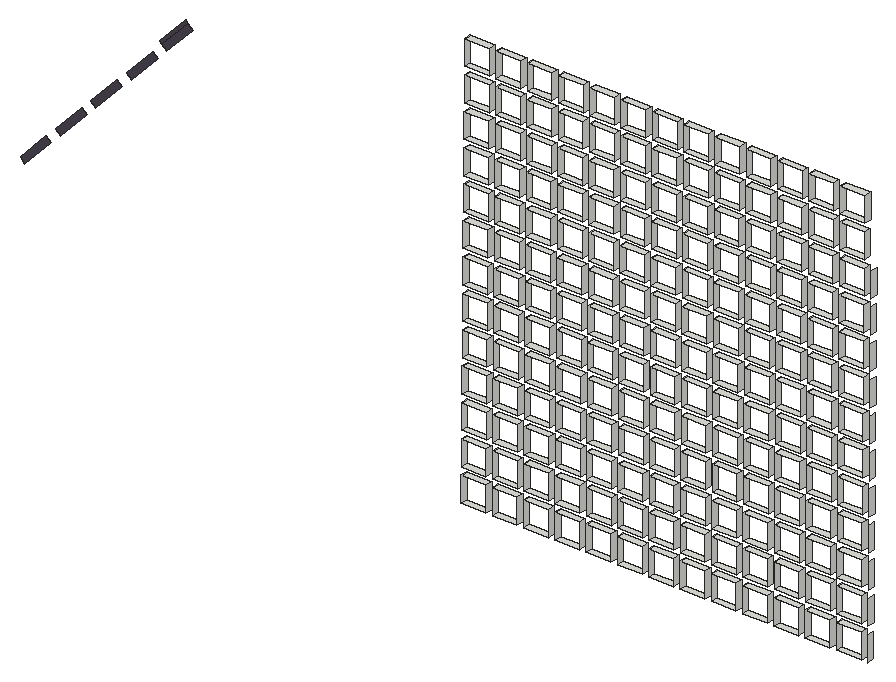
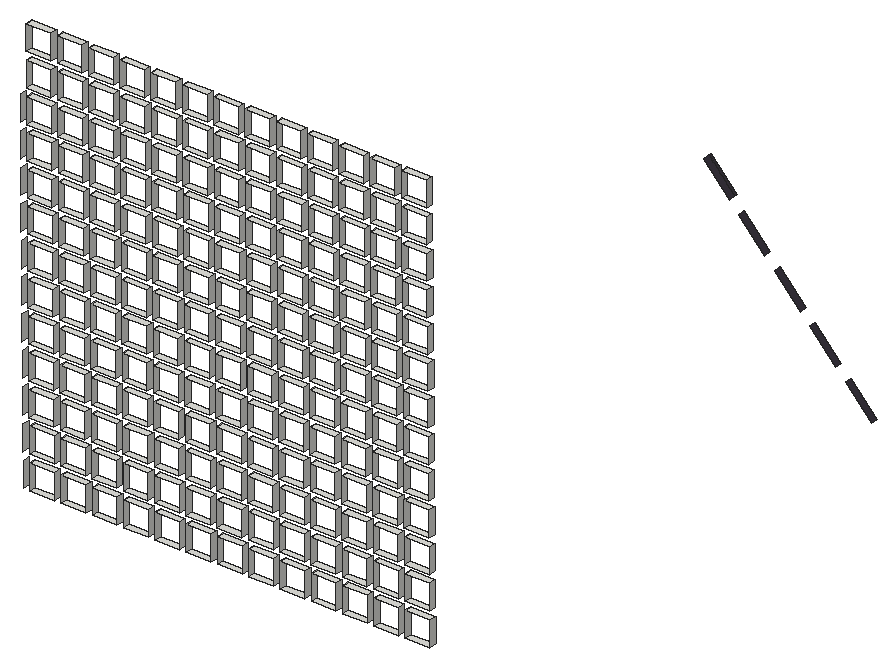
# SketchUp Ruby script. Lengths in inches.
U = 1.inch
M = Sketchup.active_model
def pt(a) = Geom::Point3d.new(a.map { |v| v * U })
def face(e, loops, mat)
  f = e.add_face(loops[0].map { |a| pt(a) })
  loops[1..].each { |l| e.add_face(l.map { |a| pt(a) }).erase! }
  f.material = f.back_material = mat if mat
  f
end
# faces: each face lists its corners as indices into pts; further lists are holes
def faces(e, pts, list, mat = nil) = list.each { |f| face(e, (f[0].is_a?(Array) ? f : [f]).map { |l| l.map { |i| pts[i] } }, mat) }
# xy, xz, yz: faces in a plane at the given z, y or x. An outline is a flat list of corners, or four numbers for a rectangle; further outlines are holes
def ring(l) = l.size == 4 ? [[l[0], l[1]], [l[2], l[1]], [l[2], l[3]], [l[0], l[3]]] : l.each_slice(2).to_a
def flat(e, list, mat, &to3) = list.each { |f| face(e, (f[0].is_a?(Array) ? f : [f]).map { |l| ring(l).map { |u, v| to3.(u, v) } }, mat) }
def xy(e, z, list, mat = nil) = flat(e, list, mat) { |x, y| [x, y, z] }
def xz(e, y, list, mat = nil) = flat(e, list, mat) { |x, z| [x, y, z] }
def yz(e, x, list, mat = nil) = flat(e, list, mat) { |y, z| [x, y, z] }
def lines(e, pts, list) = list.each { |a, b| e.add_line(pt(pts[a]), pt(pts[b])) }
# prism: a flat outline (further loops are holes) pulled along v
def prism(e, loops, v, mat = nil)
  f = face(e, loops, mat); d = Geom::Vector3d.new(v.map { |x| x * U })
  f.pushpull(f.normal.samedirection?(d) ? d.length : -d.length)
end
def box(e, o, s, mat = nil) = prism(e, [[o, [o[0] + s[0], o[1], o[2]], [o[0] + s[0], o[1] + s[1], o[2]], [o[0], o[1] + s[1], o[2]]]], [0, 0, s[2]], mat)
def at(x, y, z, deg = 0) = Geom::Transformation.translation(pt([x, y, z])) * Geom::Transformation.rotation(ORIGIN, Z_AXIS, deg.degrees)
def axes(o, x, y, z) = Geom::Transformation.new([*x, 0, *y, 0, *z, 0, *pt(o).to_a, 1])
def part(name) = M.definitions.add(name)
# library, detail: a bought-in or finely detailed component or shape, given as its bounding box
def library(name, o, s) = part(name).tap { |d| box(d.entities, o, s) }
def detail(e, o, s) = box(e.add_group.entities, o, s)
def put(e, d, t, mat = nil) = e.add_instance(d, t).tap { |i| i.material = mat if mat }
def group(e, t, mat = nil) = e.add_group.tap { |g| g.transformation = t; g.material = mat if mat }.entities
root = M.entities
M.materials.add("[Color M06]").color = [79, 71, 84]
xy(root,265.77,[[1319.26,480.14,1321.57,480.77],[1322.17,480.14,1324.48,480.77],[1325.08,480.14,1327.39,480.77],[1327.99,480.14,1330.3,480.77],[1330.9,480.14,1333.22,480.77],
  [1333.82,480.14,1336.13,480.77],[1336.73,480.14,1339.04,480.77],[1339.64,480.14,1341.95,480.77],[1342.55,480.14,1344.86,480.77],[1345.46,480.14,1347.78,480.77],
  [1348.375,480.14,1350.6875,480.77],[1351.29,480.14,1353.6,480.77],[1354.2,480.14,1356.51,480.77]])
xy(root,268.09,[[1319.26,480.14,1321.57,480.77],[1322.17,480.14,1324.48,480.77],[1325.08,480.14,1327.39,480.77],[1327.99,480.14,1330.3,480.77],[1330.9,480.14,1333.22,480.77],
  [1333.82,480.14,1336.13,480.77],[1336.73,480.14,1339.04,480.77],[1339.64,480.14,1341.95,480.77],[1342.55,480.14,1344.86,480.77],[1345.46,480.14,1347.78,480.77],
  [1348.375,480.14,1350.6875,480.77],[1351.29,480.14,1353.6,480.77],[1354.2,480.14,1356.51,480.77]])
xy(root,268.82,[[1319.28,480.14,1321.6,480.77],[1322.2,480.14,1324.51,480.77],[1325.11,480.14,1327.42,480.77],[1328.02,480.14,1330.33,480.77],[1330.93,480.14,1333.25,480.77],
  [1333.85,480.14,1336.16,480.77],[1336.76,480.14,1339.07,480.77],[1339.67,480.14,1341.98,480.77],[1342.58,480.14,1344.89,480.77],[1345.49,480.14,1347.81,480.77],
  [1348.41,480.14,1350.72,480.77],[1351.32,480.14,1353.63,480.77],[1354.23,480.14,1356.54,480.77]])
xy(root,271.13,[[1319.28,480.14,1321.6,480.77],[1322.2,480.14,1324.51,480.77],[1325.11,480.14,1327.42,480.77],[1328.02,480.14,1330.33,480.77],[1330.93,480.14,1333.25,480.77],
  [1333.85,480.14,1336.16,480.77],[1336.76,480.14,1339.07,480.77],[1339.67,480.14,1341.98,480.77],[1342.58,480.14,1344.89,480.77],[1345.49,480.14,1347.81,480.77],
  [1348.41,480.14,1350.72,480.77],[1351.32,480.14,1353.63,480.77],[1354.23,480.14,1356.54,480.77]])
xy(root,271.86,[[1319.3125,480.14,1321.625,480.77],[1322.23,480.14,1324.54,480.77],[1325.14,480.14,1327.45,480.77],[1328.05,480.14,1330.36,480.77],[1330.96,480.14,1333.27,480.77],
  [1333.875,480.14,1336.1875,480.77],[1336.79,480.14,1339.1,480.77],[1339.7,480.14,1342.01,480.77],[1342.61,480.14,1344.92,480.77],[1345.52,480.14,1347.83,480.77],
  [1348.43,480.14,1350.75,480.77],[1351.35,480.14,1353.66,480.77],[1354.26,480.14,1356.57,480.77]])
xy(root,274.17,[[1319.3125,480.14,1321.625,480.77],[1322.23,480.14,1324.54,480.77],[1325.14,480.14,1327.45,480.77],[1328.05,480.14,1330.36,480.77],[1330.96,480.14,1333.27,480.77],
  [1333.875,480.14,1336.1875,480.77],[1336.79,480.14,1339.1,480.77],[1339.7,480.14,1342.01,480.77],[1342.61,480.14,1344.92,480.77],[1345.52,480.14,1347.83,480.77],
  [1348.43,480.14,1350.75,480.77],[1351.35,480.14,1353.66,480.77],[1354.26,480.14,1356.57,480.77]])
xy(root,274.91,[[1319.34,480.14,1321.66,480.77],[1322.25,480.14,1324.57,480.77],[1325.17,480.14,1327.48,480.77],[1328.08,480.14,1330.39,480.77],[1330.99,480.14,1333.3,480.77],
  [1333.9,480.14,1336.22,480.77],[1336.82,480.14,1339.13,480.77],[1339.73,480.14,1342.04,480.77],[1342.64,480.14,1344.95,480.77],[1345.55,480.14,1347.86,480.77],
  [1348.46,480.14,1350.78,480.77],[1351.375,480.14,1353.6875,480.77],[1354.29,480.14,1356.6,480.77]])
xy(root,277.22,[[1319.34,480.14,1321.66,480.77],[1322.25,480.14,1324.57,480.77],[1325.17,480.14,1327.48,480.77],[1328.08,480.14,1330.39,480.77],[1330.99,480.14,1333.3,480.77],
  [1333.9,480.14,1336.22,480.77],[1336.82,480.14,1339.13,480.77],[1339.73,480.14,1342.04,480.77],[1342.64,480.14,1344.95,480.77],[1345.55,480.14,1347.86,480.77],
  [1348.46,480.14,1350.78,480.77],[1351.375,480.14,1353.6875,480.77],[1354.29,480.14,1356.6,480.77]])
xy(root,277.95,[[1319.37,480.14,1321.68,480.77],[1322.28,480.14,1324.6,480.77],[1325.2,480.14,1327.51,480.77],[1328.11,480.14,1330.42,480.77],[1331.02,480.14,1333.33,480.77],
  [1333.93,480.14,1336.24,480.77],[1336.84,480.14,1339.16,480.77],[1339.76,480.14,1342.07,480.77],[1342.67,480.14,1344.98,480.77],[1345.58,480.14,1347.89,480.77],
  [1348.49,480.14,1350.8,480.77],[1351.4,480.14,1353.72,480.77],[1354.32,480.14,1356.63,480.77]])
xy(root,280.26,[[1319.37,480.14,1321.68,480.77],[1322.28,480.14,1324.6,480.77],[1325.2,480.14,1327.51,480.77],[1328.11,480.14,1330.42,480.77],[1331.02,480.14,1333.33,480.77],
  [1333.93,480.14,1336.24,480.77],[1336.84,480.14,1339.16,480.77],[1339.76,480.14,1342.07,480.77],[1342.67,480.14,1344.98,480.77],[1345.58,480.14,1347.89,480.77],
  [1348.49,480.14,1350.8,480.77],[1351.4,480.14,1353.72,480.77],[1354.32,480.14,1356.63,480.77]])
xy(root,281,[[1319.4,480.14,1321.71,480.77],[1322.3125,480.14,1324.625,480.77],[1325.23,480.14,1327.54,480.77],[1328.14,480.14,1330.45,480.77],[1331.05,480.14,1333.36,480.77],
  [1333.96,480.14,1336.27,480.77],[1336.875,480.14,1339.1875,480.77],[1339.79,480.14,1342.1,480.77],[1342.7,480.14,1345.01,480.77],[1345.61,480.14,1347.92,480.77],
  [1348.52,480.14,1350.83,480.77],[1351.43,480.14,1353.75,480.77],[1354.35,480.14,1356.66,480.77]])
xy(root,283.31,[[1319.4,480.14,1321.71,480.77],[1322.3125,480.14,1324.625,480.77],[1325.23,480.14,1327.54,480.77],[1328.14,480.14,1330.45,480.77],[1331.05,480.14,1333.36,480.77],
  [1333.96,480.14,1336.27,480.77],[1336.875,480.14,1339.1875,480.77],[1339.79,480.14,1342.1,480.77],[1342.7,480.14,1345.01,480.77],[1345.61,480.14,1347.92,480.77],
  [1348.52,480.14,1350.83,480.77],[1351.43,480.14,1353.75,480.77],[1354.35,480.14,1356.66,480.77]])
xy(root,284.04,[[1319.43,480.14,1321.74,480.77],[1322.34,480.14,1324.65,480.77],[1325.25,480.14,1327.57,480.77],[1328.17,480.14,1330.48,480.77],[1331.08,480.14,1333.39,480.77],
  [1333.99,480.14,1336.3,480.77],[1336.9,480.14,1339.21,480.77],[1339.8125,480.14,1342.125,480.77],[1342.73,480.14,1345.04,480.77],[1345.64,480.14,1347.95,480.77],
  [1348.55,480.14,1350.86,480.77],[1351.46,480.14,1353.77,480.77],[1354.375,480.14,1356.6875,480.77]])
xy(root,286.35,[[1319.43,480.14,1321.74,480.77],[1322.34,480.14,1324.65,480.77],[1325.25,480.14,1327.57,480.77],[1328.17,480.14,1330.48,480.77],[1331.08,480.14,1333.39,480.77],
  [1333.99,480.14,1336.3,480.77],[1336.9,480.14,1339.21,480.77],[1339.8125,480.14,1342.125,480.77],[1342.73,480.14,1345.04,480.77],[1345.64,480.14,1347.95,480.77],
  [1348.55,480.14,1350.86,480.77],[1351.46,480.14,1353.77,480.77],[1354.375,480.14,1356.6875,480.77]])
xy(root,287.09,[[1319.46,480.14,1321.77,480.77],[1322.37,480.14,1324.68,480.77],[1325.28,480.14,1327.6,480.77],[1328.2,480.14,1330.51,480.77],[1331.11,480.14,1333.42,480.77],
  [1334.02,480.14,1336.33,480.77],[1336.93,480.14,1339.24,480.77],[1339.84,480.14,1342.16,480.77],[1342.76,480.14,1345.07,480.77],[1345.67,480.14,1347.98,480.77],
  [1348.58,480.14,1350.89,480.77],[1351.49,480.14,1353.8,480.77],[1354.4,480.14,1356.72,480.77]])
xy(root,289.4,[[1319.46,480.14,1321.77,480.77],[1322.37,480.14,1324.68,480.77],[1325.28,480.14,1327.6,480.77],[1328.2,480.14,1330.51,480.77],[1331.11,480.14,1333.42,480.77],
  [1334.02,480.14,1336.33,480.77],[1336.93,480.14,1339.24,480.77],[1339.84,480.14,1342.16,480.77],[1342.76,480.14,1345.07,480.77],[1345.67,480.14,1347.98,480.77],
  [1348.58,480.14,1350.89,480.77],[1351.49,480.14,1353.8,480.77],[1354.4,480.14,1356.72,480.77]])
xy(root,290.13,[[1319.49,480.14,1321.8,480.77],[1322.4,480.14,1324.71,480.77],[1325.3125,480.14,1327.625,480.77],[1328.22,480.14,1330.54,480.77],[1331.14,480.14,1333.45,480.77],
  [1334.05,480.14,1336.36,480.77],[1336.96,480.14,1339.27,480.77],[1339.87,480.14,1342.18,480.77],[1342.78,480.14,1345.1,480.77],[1345.7,480.14,1348.01,480.77],
  [1348.61,480.14,1350.92,480.77],[1351.52,480.14,1353.83,480.77],[1354.43,480.14,1356.74,480.77]])
xy(root,292.44,[[1319.49,480.14,1321.8,480.77],[1322.4,480.14,1324.71,480.77],[1325.3125,480.14,1327.625,480.77],[1328.22,480.14,1330.54,480.77],[1331.14,480.14,1333.45,480.77],
  [1334.05,480.14,1336.36,480.77],[1336.96,480.14,1339.27,480.77],[1339.87,480.14,1342.18,480.77],[1342.78,480.14,1345.1,480.77],[1345.7,480.14,1348.01,480.77],
  [1348.61,480.14,1350.92,480.77],[1351.52,480.14,1353.83,480.77],[1354.43,480.14,1356.74,480.77]])
xy(root,293.18,[[1319.52,480.14,1321.83,480.77],[1322.43,480.14,1324.74,480.77],[1325.34,480.14,1327.65,480.77],[1328.25,480.14,1330.57,480.77],[1331.17,480.14,1333.48,480.77],
  [1334.08,480.14,1336.39,480.77],[1336.99,480.14,1339.3,480.77],[1339.9,480.14,1342.21,480.77],[1342.8125,480.14,1345.125,480.77],[1345.73,480.14,1348.04,480.77],
  [1348.64,480.14,1350.95,480.77],[1351.55,480.14,1353.86,480.77],[1354.46,480.14,1356.77,480.77]])
xy(root,295.49,[[1319.52,480.14,1321.83,480.77],[1322.43,480.14,1324.74,480.77],[1325.34,480.14,1327.65,480.77],[1328.25,480.14,1330.57,480.77],[1331.17,480.14,1333.48,480.77],
  [1334.08,480.14,1336.39,480.77],[1336.99,480.14,1339.3,480.77],[1339.9,480.14,1342.21,480.77],[1342.8125,480.14,1345.125,480.77],[1345.73,480.14,1348.04,480.77],
  [1348.64,480.14,1350.95,480.77],[1351.55,480.14,1353.86,480.77],[1354.46,480.14,1356.77,480.77]])
xy(root,296.22,[[1319.55,480.14,1321.86,480.77],[1322.46,480.14,1324.77,480.77],[1325.37,480.14,1327.68,480.77],[1328.28,480.14,1330.59,480.77],[1331.19,480.14,1333.51,480.77],
  [1334.11,480.14,1336.42,480.77],[1337.02,480.14,1339.33,480.77],[1339.93,480.14,1342.24,480.77],[1342.84,480.14,1345.15,480.77],[1345.75,480.14,1348.07,480.77],
  [1348.67,480.14,1350.98,480.77],[1351.58,480.14,1353.89,480.77],[1354.49,480.14,1356.8,480.77]])
xy(root,298.53,[[1319.55,480.14,1321.86,480.77],[1322.46,480.14,1324.77,480.77],[1325.37,480.14,1327.68,480.77],[1328.28,480.14,1330.59,480.77],[1331.19,480.14,1333.51,480.77],
  [1334.11,480.14,1336.42,480.77],[1337.02,480.14,1339.33,480.77],[1339.93,480.14,1342.24,480.77],[1342.84,480.14,1345.15,480.77],[1345.75,480.14,1348.07,480.77],
  [1348.67,480.14,1350.98,480.77],[1351.58,480.14,1353.89,480.77],[1354.49,480.14,1356.8,480.77]])
xy(root,299.27,[[1319.57,480.14,1321.89,480.77],[1322.49,480.14,1324.8,480.77],[1325.4,480.14,1327.71,480.77],[1328.3125,480.14,1330.625,480.77],[1331.22,480.14,1333.54,480.77],
  [1334.14,480.14,1336.45,480.77],[1337.05,480.14,1339.36,480.77],[1339.96,480.14,1342.27,480.77],[1342.87,480.14,1345.18,480.77],[1345.78,480.14,1348.1,480.77],
  [1348.7,480.14,1351.01,480.77],[1351.61,480.14,1353.92,480.77],[1354.52,480.14,1356.83,480.77]])
xy(root,301.58,[[1319.57,480.14,1321.89,480.77],[1322.49,480.14,1324.8,480.77],[1325.4,480.14,1327.71,480.77],[1328.3125,480.14,1330.625,480.77],[1331.22,480.14,1333.54,480.77],
  [1334.14,480.14,1336.45,480.77],[1337.05,480.14,1339.36,480.77],[1339.96,480.14,1342.27,480.77],[1342.87,480.14,1345.18,480.77],[1345.78,480.14,1348.1,480.77],
  [1348.7,480.14,1351.01,480.77],[1351.61,480.14,1353.92,480.77],[1354.52,480.14,1356.83,480.77]])
xy(root,302.31,[[1319.6,480.14,1321.92,480.77],[1322.52,480.14,1324.83,480.77],[1325.43,480.14,1327.74,480.77],[1328.34,480.14,1330.65,480.77],[1331.25,480.14,1333.56,480.77],
  [1334.16,480.14,1336.48,480.77],[1337.08,480.14,1339.39,480.77],[1339.99,480.14,1342.3,480.77],[1342.9,480.14,1345.21,480.77],[1345.8125,480.14,1348.125,480.77],
  [1348.72,480.14,1351.04,480.77],[1351.64,480.14,1353.95,480.77],[1354.55,480.14,1356.86,480.77]])
xy(root,304.62,[[1319.6,480.14,1321.92,480.77],[1322.52,480.14,1324.83,480.77],[1325.43,480.14,1327.74,480.77],[1328.34,480.14,1330.65,480.77],[1331.25,480.14,1333.56,480.77],
  [1334.16,480.14,1336.48,480.77],[1337.08,480.14,1339.39,480.77],[1339.99,480.14,1342.3,480.77],[1342.9,480.14,1345.21,480.77],[1345.8125,480.14,1348.125,480.77],
  [1348.72,480.14,1351.04,480.77],[1351.64,480.14,1353.95,480.77],[1354.55,480.14,1356.86,480.77]])
xz(root,467.1875,[[1289.04,289.13,1291.46,291.7,1291.01,292.13,1288.59,289.56],[1292.34,292.64,1294.76,295.21,1294.3,295.64,1291.88,293.0625],[1295.64,296.14,1298.06,298.71,1297.6,299.14,1295.18,296.57],[1298.9375,299.64,1301.36,302.22,1300.9,302.64,1298.48,300.07],[1302.23,303.15,1304.66,305.72,1304.2,306.15,1301.78,303.58],
  [1301.78,303.58,1304.2,306.15,1303.97,306.36,1301.55,303.79]],"[Color M06]")
yz(root,1319.26,[[480.14,265.77,480.77,268.09]])
yz(root,1319.28,[[480.14,268.82,480.77,271.13]])
yz(root,1319.3125,[[480.14,271.86,480.77,274.17]])
yz(root,1319.34,[[480.14,274.91,480.77,277.22]])
yz(root,1319.37,[[480.14,277.95,480.77,280.26]])
yz(root,1319.4,[[480.14,281,480.77,283.31]])
yz(root,1319.43,[[480.14,284.04,480.77,286.35]])
yz(root,1319.46,[[480.14,287.09,480.77,289.4]])
yz(root,1319.49,[[480.14,290.13,480.77,292.44]])
yz(root,1319.52,[[480.14,293.18,480.77,295.49]])
yz(root,1319.55,[[480.14,296.22,480.77,298.53]])
yz(root,1319.57,[[480.14,299.27,480.77,301.58]])
yz(root,1319.6,[[480.14,302.31,480.77,304.62]])
yz(root,1321.57,[[480.14,265.77,480.77,268.09]])
yz(root,1321.6,[[480.14,268.82,480.77,271.13]])
yz(root,1321.625,[[480.14,271.86,480.77,274.17]])
yz(root,1321.66,[[480.14,274.91,480.77,277.22]])
yz(root,1321.68,[[480.14,277.95,480.77,280.26]])
yz(root,1321.71,[[480.14,281,480.77,283.31]])
yz(root,1321.74,[[480.14,284.04,480.77,286.35]])
yz(root,1321.77,[[480.14,287.09,480.77,289.4]])
yz(root,1321.8,[[480.14,290.13,480.77,292.44]])
yz(root,1321.83,[[480.14,293.18,480.77,295.49]])
yz(root,1321.86,[[480.14,296.22,480.77,298.53]])
yz(root,1321.89,[[480.14,299.27,480.77,301.58]])
yz(root,1321.92,[[480.14,302.31,480.77,304.62]])
yz(root,1322.17,[[480.14,265.77,480.77,268.09]])
yz(root,1322.2,[[480.14,268.82,480.77,271.13]])
yz(root,1322.23,[[480.14,271.86,480.77,274.17]])
yz(root,1322.25,[[480.14,274.91,480.77,277.22]])
yz(root,1322.28,[[480.14,277.95,480.77,280.26]])
yz(root,1322.3125,[[480.14,281,480.77,283.31]])
yz(root,1322.34,[[480.14,284.04,480.77,286.35]])
yz(root,1322.37,[[480.14,287.09,480.77,289.4]])
yz(root,1322.4,[[480.14,290.13,480.77,292.44]])
yz(root,1322.43,[[480.14,293.18,480.77,295.49]])
yz(root,1322.46,[[480.14,296.22,480.77,298.53]])
yz(root,1322.49,[[480.14,299.27,480.77,301.58]])
yz(root,1322.52,[[480.14,302.31,480.77,304.62]])
yz(root,1324.48,[[480.14,265.77,480.77,268.09]])
yz(root,1324.51,[[480.14,268.82,480.77,271.13]])
yz(root,1324.54,[[480.14,271.86,480.77,274.17]])
yz(root,1324.57,[[480.14,274.91,480.77,277.22]])
yz(root,1324.6,[[480.14,277.95,480.77,280.26]])
yz(root,1324.625,[[480.14,281,480.77,283.31]])
yz(root,1324.65,[[480.14,284.04,480.77,286.35]])
yz(root,1324.68,[[480.14,287.09,480.77,289.4]])
yz(root,1324.71,[[480.14,290.13,480.77,292.44]])
yz(root,1324.74,[[480.14,293.18,480.77,295.49]])
yz(root,1324.77,[[480.14,296.22,480.77,298.53]])
yz(root,1324.8,[[480.14,299.27,480.77,301.58]])
yz(root,1324.83,[[480.14,302.31,480.77,304.62]])
yz(root,1325.08,[[480.14,265.77,480.77,268.09]])
yz(root,1325.11,[[480.14,268.82,480.77,271.13]])
yz(root,1325.14,[[480.14,271.86,480.77,274.17]])
yz(root,1325.17,[[480.14,274.91,480.77,277.22]])
yz(root,1325.2,[[480.14,277.95,480.77,280.26]])
yz(root,1325.23,[[480.14,281,480.77,283.31]])
yz(root,1325.25,[[480.14,284.04,480.77,286.35]])
yz(root,1325.28,[[480.14,287.09,480.77,289.4]])
yz(root,1325.3125,[[480.14,290.13,480.77,292.44]])
yz(root,1325.34,[[480.14,293.18,480.77,295.49]])
yz(root,1325.37,[[480.14,296.22,480.77,298.53]])
yz(root,1325.4,[[480.14,299.27,480.77,301.58]])
yz(root,1325.43,[[480.14,302.31,480.77,304.62]])
yz(root,1327.39,[[480.14,265.77,480.77,268.09]])
yz(root,1327.42,[[480.14,268.82,480.77,271.13]])
yz(root,1327.45,[[480.14,271.86,480.77,274.17]])
yz(root,1327.48,[[480.14,274.91,480.77,277.22]])
yz(root,1327.51,[[480.14,277.95,480.77,280.26]])
yz(root,1327.54,[[480.14,281,480.77,283.31]])
yz(root,1327.57,[[480.14,284.04,480.77,286.35]])
yz(root,1327.6,[[480.14,287.09,480.77,289.4]])
yz(root,1327.625,[[480.14,290.13,480.77,292.44]])
yz(root,1327.65,[[480.14,293.18,480.77,295.49]])
yz(root,1327.68,[[480.14,296.22,480.77,298.53]])
yz(root,1327.71,[[480.14,299.27,480.77,301.58]])
yz(root,1327.74,[[480.14,302.31,480.77,304.62]])
yz(root,1327.99,[[480.14,265.77,480.77,268.09]])
yz(root,1328.02,[[480.14,268.82,480.77,271.13]])
yz(root,1328.05,[[480.14,271.86,480.77,274.17]])
yz(root,1328.08,[[480.14,274.91,480.77,277.22]])
yz(root,1328.11,[[480.14,277.95,480.77,280.26]])
yz(root,1328.14,[[480.14,281,480.77,283.31]])
yz(root,1328.17,[[480.14,284.04,480.77,286.35]])
yz(root,1328.2,[[480.14,287.09,480.77,289.4]])
yz(root,1328.22,[[480.14,290.13,480.77,292.44]])
yz(root,1328.25,[[480.14,293.18,480.77,295.49]])
yz(root,1328.28,[[480.14,296.22,480.77,298.53]])
yz(root,1328.3125,[[480.14,299.27,480.77,301.58]])
yz(root,1328.34,[[480.14,302.31,480.77,304.62]])
yz(root,1330.3,[[480.14,265.77,480.77,268.09]])
yz(root,1330.33,[[480.14,268.82,480.77,271.13]])
yz(root,1330.36,[[480.14,271.86,480.77,274.17]])
yz(root,1330.39,[[480.14,274.91,480.77,277.22]])
yz(root,1330.42,[[480.14,277.95,480.77,280.26]])
yz(root,1330.45,[[480.14,281,480.77,283.31]])
yz(root,1330.48,[[480.14,284.04,480.77,286.35]])
yz(root,1330.51,[[480.14,287.09,480.77,289.4]])
yz(root,1330.54,[[480.14,290.13,480.77,292.44]])
yz(root,1330.57,[[480.14,293.18,480.77,295.49]])
yz(root,1330.59,[[480.14,296.22,480.77,298.53]])
yz(root,1330.625,[[480.14,299.27,480.77,301.58]])
yz(root,1330.65,[[480.14,302.31,480.77,304.62]])
yz(root,1330.9,[[480.14,265.77,480.77,268.09]])
yz(root,1330.93,[[480.14,268.82,480.77,271.13]])
yz(root,1330.96,[[480.14,271.86,480.77,274.17]])
yz(root,1330.99,[[480.14,274.91,480.77,277.22]])
yz(root,1331.02,[[480.14,277.95,480.77,280.26]])
yz(root,1331.05,[[480.14,281,480.77,283.31]])
yz(root,1331.08,[[480.14,284.04,480.77,286.35]])
yz(root,1331.11,[[480.14,287.09,480.77,289.4]])
yz(root,1331.14,[[480.14,290.13,480.77,292.44]])
yz(root,1331.17,[[480.14,293.18,480.77,295.49]])
yz(root,1331.19,[[480.14,296.22,480.77,298.53]])
yz(root,1331.22,[[480.14,299.27,480.77,301.58]])
yz(root,1331.25,[[480.14,302.31,480.77,304.62]])
yz(root,1333.22,[[480.14,265.77,480.77,268.09]])
yz(root,1333.25,[[480.14,268.82,480.77,271.13]])
yz(root,1333.27,[[480.14,271.86,480.77,274.17]])
yz(root,1333.3,[[480.14,274.91,480.77,277.22]])
yz(root,1333.33,[[480.14,277.95,480.77,280.26]])
yz(root,1333.36,[[480.14,281,480.77,283.31]])
yz(root,1333.39,[[480.14,284.04,480.77,286.35]])
yz(root,1333.42,[[480.14,287.09,480.77,289.4]])
yz(root,1333.45,[[480.14,290.13,480.77,292.44]])
yz(root,1333.48,[[480.14,293.18,480.77,295.49]])
yz(root,1333.51,[[480.14,296.22,480.77,298.53]])
yz(root,1333.54,[[480.14,299.27,480.77,301.58]])
yz(root,1333.56,[[480.14,302.31,480.77,304.62]])
yz(root,1333.82,[[480.14,265.77,480.77,268.09]])
yz(root,1333.85,[[480.14,268.82,480.77,271.13]])
yz(root,1333.875,[[480.14,271.86,480.77,274.17]])
yz(root,1333.9,[[480.14,274.91,480.77,277.22]])
yz(root,1333.93,[[480.14,277.95,480.77,280.26]])
yz(root,1333.96,[[480.14,281,480.77,283.31]])
yz(root,1333.99,[[480.14,284.04,480.77,286.35]])
yz(root,1334.02,[[480.14,287.09,480.77,289.4]])
yz(root,1334.05,[[480.14,290.13,480.77,292.44]])
yz(root,1334.08,[[480.14,293.18,480.77,295.49]])
yz(root,1334.11,[[480.14,296.22,480.77,298.53]])
yz(root,1334.14,[[480.14,299.27,480.77,301.58]])
yz(root,1334.16,[[480.14,302.31,480.77,304.62]])
yz(root,1336.13,[[480.14,265.77,480.77,268.09]])
yz(root,1336.16,[[480.14,268.82,480.77,271.13]])
yz(root,1336.1875,[[480.14,271.86,480.77,274.17]])
yz(root,1336.22,[[480.14,274.91,480.77,277.22]])
yz(root,1336.24,[[480.14,277.95,480.77,280.26]])
yz(root,1336.27,[[480.14,281,480.77,283.31]])
yz(root,1336.3,[[480.14,284.04,480.77,286.35]])
yz(root,1336.33,[[480.14,287.09,480.77,289.4]])
yz(root,1336.36,[[480.14,290.13,480.77,292.44]])
yz(root,1336.39,[[480.14,293.18,480.77,295.49]])
yz(root,1336.42,[[480.14,296.22,480.77,298.53]])
yz(root,1336.45,[[480.14,299.27,480.77,301.58]])
yz(root,1336.48,[[480.14,302.31,480.77,304.62]])
yz(root,1336.73,[[480.14,265.77,480.77,268.09]])
yz(root,1336.76,[[480.14,268.82,480.77,271.13]])
yz(root,1336.79,[[480.14,271.86,480.77,274.17]])
yz(root,1336.82,[[480.14,274.91,480.77,277.22]])
yz(root,1336.84,[[480.14,277.95,480.77,280.26]])
yz(root,1336.875,[[480.14,281,480.77,283.31]])
yz(root,1336.9,[[480.14,284.04,480.77,286.35]])
yz(root,1336.93,[[480.14,287.09,480.77,289.4]])
yz(root,1336.96,[[480.14,290.13,480.77,292.44]])
yz(root,1336.99,[[480.14,293.18,480.77,295.49]])
yz(root,1337.02,[[480.14,296.22,480.77,298.53]])
yz(root,1337.05,[[480.14,299.27,480.77,301.58]])
yz(root,1337.08,[[480.14,302.31,480.77,304.62]])
yz(root,1339.04,[[480.14,265.77,480.77,268.09]])
yz(root,1339.07,[[480.14,268.82,480.77,271.13]])
yz(root,1339.1,[[480.14,271.86,480.77,274.17]])
yz(root,1339.13,[[480.14,274.91,480.77,277.22]])
yz(root,1339.16,[[480.14,277.95,480.77,280.26]])
yz(root,1339.1875,[[480.14,281,480.77,283.31]])
yz(root,1339.21,[[480.14,284.04,480.77,286.35]])
yz(root,1339.24,[[480.14,287.09,480.77,289.4]])
yz(root,1339.27,[[480.14,290.13,480.77,292.44]])
yz(root,1339.3,[[480.14,293.18,480.77,295.49]])
yz(root,1339.33,[[480.14,296.22,480.77,298.53]])
yz(root,1339.36,[[480.14,299.27,480.77,301.58]])
yz(root,1339.39,[[480.14,302.31,480.77,304.62]])
yz(root,1339.64,[[480.14,265.77,480.77,268.09]])
yz(root,1339.67,[[480.14,268.82,480.77,271.13]])
yz(root,1339.7,[[480.14,271.86,480.77,274.17]])
yz(root,1339.73,[[480.14,274.91,480.77,277.22]])
yz(root,1339.76,[[480.14,277.95,480.77,280.26]])
yz(root,1339.79,[[480.14,281,480.77,283.31]])
yz(root,1339.8125,[[480.14,284.04,480.77,286.35]])
yz(root,1339.84,[[480.14,287.09,480.77,289.4]])
yz(root,1339.87,[[480.14,290.13,480.77,292.44]])
yz(root,1339.9,[[480.14,293.18,480.77,295.49]])
yz(root,1339.93,[[480.14,296.22,480.77,298.53]])
yz(root,1339.96,[[480.14,299.27,480.77,301.58]])
yz(root,1339.99,[[480.14,302.31,480.77,304.62]])
yz(root,1341.95,[[480.14,265.77,480.77,268.09]])
yz(root,1341.98,[[480.14,268.82,480.77,271.13]])
yz(root,1342.01,[[480.14,271.86,480.77,274.17]])
yz(root,1342.04,[[480.14,274.91,480.77,277.22]])
yz(root,1342.07,[[480.14,277.95,480.77,280.26]])
yz(root,1342.1,[[480.14,281,480.77,283.31]])
yz(root,1342.125,[[480.14,284.04,480.77,286.35]])
yz(root,1342.16,[[480.14,287.09,480.77,289.4]])
yz(root,1342.18,[[480.14,290.13,480.77,292.44]])
yz(root,1342.21,[[480.14,293.18,480.77,295.49]])
yz(root,1342.24,[[480.14,296.22,480.77,298.53]])
yz(root,1342.27,[[480.14,299.27,480.77,301.58]])
yz(root,1342.3,[[480.14,302.31,480.77,304.62]])
yz(root,1342.55,[[480.14,265.77,480.77,268.09]])
yz(root,1342.58,[[480.14,268.82,480.77,271.13]])
yz(root,1342.61,[[480.14,271.86,480.77,274.17]])
yz(root,1342.64,[[480.14,274.91,480.77,277.22]])
yz(root,1342.67,[[480.14,277.95,480.77,280.26]])
yz(root,1342.7,[[480.14,281,480.77,283.31]])
yz(root,1342.73,[[480.14,284.04,480.77,286.35]])
yz(root,1342.76,[[480.14,287.09,480.77,289.4]])
yz(root,1342.78,[[480.14,290.13,480.77,292.44]])
yz(root,1342.8125,[[480.14,293.18,480.77,295.49]])
yz(root,1342.84,[[480.14,296.22,480.77,298.53]])
yz(root,1342.87,[[480.14,299.27,480.77,301.58]])
yz(root,1342.9,[[480.14,302.31,480.77,304.62]])
yz(root,1344.86,[[480.14,265.77,480.77,268.09]])
yz(root,1344.89,[[480.14,268.82,480.77,271.13]])
yz(root,1344.92,[[480.14,271.86,480.77,274.17]])
yz(root,1344.95,[[480.14,274.91,480.77,277.22]])
yz(root,1344.98,[[480.14,277.95,480.77,280.26]])
yz(root,1345.01,[[480.14,281,480.77,283.31]])
yz(root,1345.04,[[480.14,284.04,480.77,286.35]])
yz(root,1345.07,[[480.14,287.09,480.77,289.4]])
yz(root,1345.1,[[480.14,290.13,480.77,292.44]])
yz(root,1345.125,[[480.14,293.18,480.77,295.49]])
yz(root,1345.15,[[480.14,296.22,480.77,298.53]])
yz(root,1345.18,[[480.14,299.27,480.77,301.58]])
yz(root,1345.21,[[480.14,302.31,480.77,304.62]])
yz(root,1345.46,[[480.14,265.77,480.77,268.09]])
yz(root,1345.49,[[480.14,268.82,480.77,271.13]])
yz(root,1345.52,[[480.14,271.86,480.77,274.17]])
yz(root,1345.55,[[480.14,274.91,480.77,277.22]])
yz(root,1345.58,[[480.14,277.95,480.77,280.26]])
yz(root,1345.61,[[480.14,281,480.77,283.31]])
yz(root,1345.64,[[480.14,284.04,480.77,286.35]])
yz(root,1345.67,[[480.14,287.09,480.77,289.4]])
yz(root,1345.7,[[480.14,290.13,480.77,292.44]])
yz(root,1345.73,[[480.14,293.18,480.77,295.49]])
yz(root,1345.75,[[480.14,296.22,480.77,298.53]])
yz(root,1345.78,[[480.14,299.27,480.77,301.58]])
yz(root,1345.8125,[[480.14,302.31,480.77,304.62]])
yz(root,1347.78,[[480.14,265.77,480.77,268.09]])
yz(root,1347.81,[[480.14,268.82,480.77,271.13]])
yz(root,1347.83,[[480.14,271.86,480.77,274.17]])
yz(root,1347.86,[[480.14,274.91,480.77,277.22]])
yz(root,1347.89,[[480.14,277.95,480.77,280.26]])
yz(root,1347.92,[[480.14,281,480.77,283.31]])
yz(root,1347.95,[[480.14,284.04,480.77,286.35]])
yz(root,1347.98,[[480.14,287.09,480.77,289.4]])
yz(root,1348.01,[[480.14,290.13,480.77,292.44]])
yz(root,1348.04,[[480.14,293.18,480.77,295.49]])
yz(root,1348.07,[[480.14,296.22,480.77,298.53]])
yz(root,1348.1,[[480.14,299.27,480.77,301.58]])
yz(root,1348.125,[[480.14,302.31,480.77,304.62]])
yz(root,1348.375,[[480.14,265.77,480.77,268.09]])
yz(root,1348.41,[[480.14,268.82,480.77,271.13]])
yz(root,1348.43,[[480.14,271.86,480.77,274.17]])
yz(root,1348.46,[[480.14,274.91,480.77,277.22]])
yz(root,1348.49,[[480.14,277.95,480.77,280.26]])
yz(root,1348.52,[[480.14,281,480.77,283.31]])
yz(root,1348.55,[[480.14,284.04,480.77,286.35]])
yz(root,1348.58,[[480.14,287.09,480.77,289.4]])
yz(root,1348.61,[[480.14,290.13,480.77,292.44]])
yz(root,1348.64,[[480.14,293.18,480.77,295.49]])
yz(root,1348.67,[[480.14,296.22,480.77,298.53]])
yz(root,1348.7,[[480.14,299.27,480.77,301.58]])
yz(root,1348.72,[[480.14,302.31,480.77,304.62]])
yz(root,1350.6875,[[480.14,265.77,480.77,268.09]])
yz(root,1350.72,[[480.14,268.82,480.77,271.13]])
yz(root,1350.75,[[480.14,271.86,480.77,274.17]])
yz(root,1350.78,[[480.14,274.91,480.77,277.22]])
yz(root,1350.8,[[480.14,277.95,480.77,280.26]])
yz(root,1350.83,[[480.14,281,480.77,283.31]])
yz(root,1350.86,[[480.14,284.04,480.77,286.35]])
yz(root,1350.89,[[480.14,287.09,480.77,289.4]])
yz(root,1350.92,[[480.14,290.13,480.77,292.44]])
yz(root,1350.95,[[480.14,293.18,480.77,295.49]])
yz(root,1350.98,[[480.14,296.22,480.77,298.53]])
yz(root,1351.01,[[480.14,299.27,480.77,301.58]])
yz(root,1351.04,[[480.14,302.31,480.77,304.62]])
yz(root,1351.29,[[480.14,265.77,480.77,268.09]])
yz(root,1351.32,[[480.14,268.82,480.77,271.13]])
yz(root,1351.35,[[480.14,271.86,480.77,274.17]])
yz(root,1351.375,[[480.14,274.91,480.77,277.22]])
yz(root,1351.4,[[480.14,277.95,480.77,280.26]])
yz(root,1351.43,[[480.14,281,480.77,283.31]])
yz(root,1351.46,[[480.14,284.04,480.77,286.35]])
yz(root,1351.49,[[480.14,287.09,480.77,289.4]])
yz(root,1351.52,[[480.14,290.13,480.77,292.44]])
yz(root,1351.55,[[480.14,293.18,480.77,295.49]])
yz(root,1351.58,[[480.14,296.22,480.77,298.53]])
yz(root,1351.61,[[480.14,299.27,480.77,301.58]])
yz(root,1351.64,[[480.14,302.31,480.77,304.62]])
yz(root,1353.6,[[480.14,265.77,480.77,268.09]])
yz(root,1353.63,[[480.14,268.82,480.77,271.13]])
yz(root,1353.66,[[480.14,271.86,480.77,274.17]])
yz(root,1353.6875,[[480.14,274.91,480.77,277.22]])
yz(root,1353.72,[[480.14,277.95,480.77,280.26]])
yz(root,1353.75,[[480.14,281,480.77,283.31]])
yz(root,1353.77,[[480.14,284.04,480.77,286.35]])
yz(root,1353.8,[[480.14,287.09,480.77,289.4]])
yz(root,1353.83,[[480.14,290.13,480.77,292.44]])
yz(root,1353.86,[[480.14,293.18,480.77,295.49]])
yz(root,1353.89,[[480.14,296.22,480.77,298.53]])
yz(root,1353.92,[[480.14,299.27,480.77,301.58]])
yz(root,1353.95,[[480.14,302.31,480.77,304.62]])
yz(root,1354.2,[[480.14,265.77,480.77,268.09]])
yz(root,1354.23,[[480.14,268.82,480.77,271.13]])
yz(root,1354.26,[[480.14,271.86,480.77,274.17]])
yz(root,1354.29,[[480.14,274.91,480.77,277.22]])
yz(root,1354.32,[[480.14,277.95,480.77,280.26]])
yz(root,1354.35,[[480.14,281,480.77,283.31]])
yz(root,1354.375,[[480.14,284.04,480.77,286.35]])
yz(root,1354.4,[[480.14,287.09,480.77,289.4]])
yz(root,1354.43,[[480.14,290.13,480.77,292.44]])
yz(root,1354.46,[[480.14,293.18,480.77,295.49]])
yz(root,1354.49,[[480.14,296.22,480.77,298.53]])
yz(root,1354.52,[[480.14,299.27,480.77,301.58]])
yz(root,1354.55,[[480.14,302.31,480.77,304.62]])
yz(root,1356.51,[[480.14,265.77,480.77,268.09]])
yz(root,1356.54,[[480.14,268.82,480.77,271.13]])
yz(root,1356.57,[[480.14,271.86,480.77,274.17]])
yz(root,1356.6,[[480.14,274.91,480.77,277.22]])
yz(root,1356.63,[[480.14,277.95,480.77,280.26]])
yz(root,1356.66,[[480.14,281,480.77,283.31]])
yz(root,1356.6875,[[480.14,284.04,480.77,286.35]])
yz(root,1356.72,[[480.14,287.09,480.77,289.4]])
yz(root,1356.74,[[480.14,290.13,480.77,292.44]])
yz(root,1356.77,[[480.14,293.18,480.77,295.49]])
yz(root,1356.8,[[480.14,296.22,480.77,298.53]])
yz(root,1356.83,[[480.14,299.27,480.77,301.58]])
yz(root,1356.86,[[480.14,302.31,480.77,304.62]])
yz(root,1357.11,[[480.14,265.77,480.77,268.09]])
yz(root,1357.14,[[480.14,268.82,480.77,271.13]])
yz(root,1357.17,[[480.14,271.86,480.77,274.17]])
yz(root,1357.2,[[480.14,274.91,480.77,277.22]])
yz(root,1357.23,[[480.14,277.95,480.77,280.26]])
yz(root,1357.26,[[480.14,281,480.77,283.31]])
yz(root,1357.29,[[480.14,284.04,480.77,286.35]])
yz(root,1357.32,[[480.14,287.09,480.77,289.4]])
yz(root,1357.34,[[480.14,290.13,480.77,292.44]])
yz(root,1357.375,[[480.14,293.18,480.77,295.49]])
yz(root,1357.4,[[480.14,296.22,480.77,298.53]])
